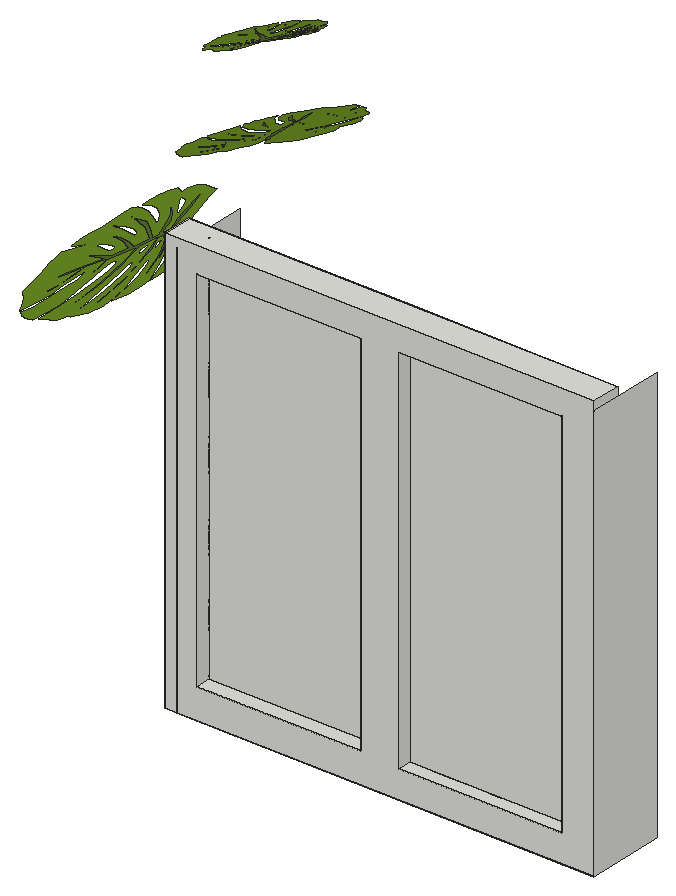
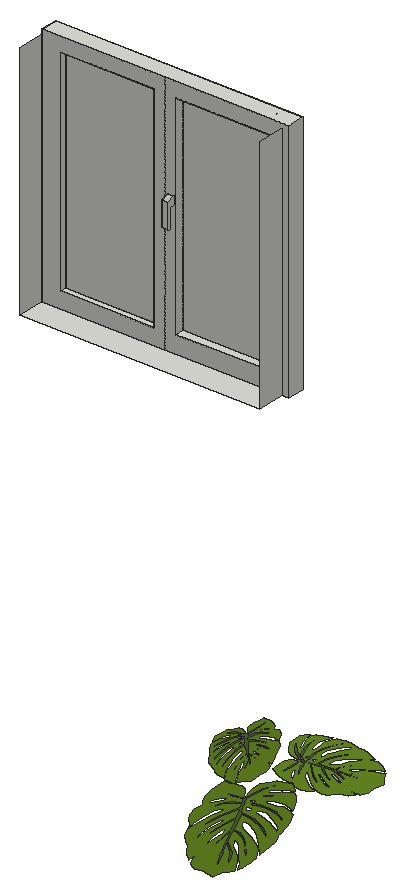
# SketchUp Ruby script. Lengths in inches.
U = 1.inch
M = Sketchup.active_model
def pt(a) = Geom::Point3d.new(a.map { |v| v * U })
def face(e, loops, mat)
  f = e.add_face(loops[0].map { |a| pt(a) })
  loops[1..].each { |l| e.add_face(l.map { |a| pt(a) }).erase! }
  f.material = f.back_material = mat if mat
  f
end
# faces: each face lists its corners as indices into pts; further lists are holes
def faces(e, pts, list, mat = nil) = list.each { |f| face(e, (f[0].is_a?(Array) ? f : [f]).map { |l| l.map { |i| pts[i] } }, mat) }
# xy, xz, yz: faces in a plane at the given z, y or x. An outline is a flat list of corners, or four numbers for a rectangle; further outlines are holes
def ring(l) = l.size == 4 ? [[l[0], l[1]], [l[2], l[1]], [l[2], l[3]], [l[0], l[3]]] : l.each_slice(2).to_a
def flat(e, list, mat, &to3) = list.each { |f| face(e, (f[0].is_a?(Array) ? f : [f]).map { |l| ring(l).map { |u, v| to3.(u, v) } }, mat) }
def xy(e, z, list, mat = nil) = flat(e, list, mat) { |x, y| [x, y, z] }
def xz(e, y, list, mat = nil) = flat(e, list, mat) { |x, z| [x, y, z] }
def yz(e, x, list, mat = nil) = flat(e, list, mat) { |y, z| [x, y, z] }
def lines(e, pts, list) = list.each { |a, b| e.add_line(pt(pts[a]), pt(pts[b])) }
# prism: a flat outline (further loops are holes) pulled along v
def prism(e, loops, v, mat = nil)
  f = face(e, loops, mat); d = Geom::Vector3d.new(v.map { |x| x * U })
  f.pushpull(f.normal.samedirection?(d) ? d.length : -d.length)
end
def box(e, o, s, mat = nil) = prism(e, [[o, [o[0] + s[0], o[1], o[2]], [o[0] + s[0], o[1] + s[1], o[2]], [o[0], o[1] + s[1], o[2]]]], [0, 0, s[2]], mat)
def at(x, y, z, deg = 0) = Geom::Transformation.translation(pt([x, y, z])) * Geom::Transformation.rotation(ORIGIN, Z_AXIS, deg.degrees)
def axes(o, x, y, z) = Geom::Transformation.new([*x, 0, *y, 0, *z, 0, *pt(o).to_a, 1])
def part(name) = M.definitions.add(name)
# library, detail: a bought-in or finely detailed component or shape, given as its bounding box
def library(name, o, s) = part(name).tap { |d| box(d.entities, o, s) }
def detail(e, o, s) = box(e.add_group.entities, o, s)
def put(e, d, t, mat = nil) = e.add_instance(d, t).tap { |i| i.material = mat if mat }
def group(e, t, mat = nil) = e.add_group.tap { |g| g.transformation = t; g.material = mat if mat }.entities
root = M.entities
M.materials.add("[0059_DarkOliveGreen]").color = [85, 107, 47]
M.materials.add("[0061_OliveDrab]").color = [107, 142, 35]
c1 = part("Window")
xy(c1.entities,31.72,[[-0.78,88.6,2.72,128.1]])
xy(c1.entities,34.95,[[-0.78,91.53,0.84,106.59],[0.84,91.53,1.05,97.58],[1.05,91.53,1.42,106.59],[1.42,91.53,2.72,106.59],[0.84,97.58,1.05,98.18],
  [0.84,98.18,1.05,106.59]])
xy(c1.entities,35.27,[[-0.78,110.09,0.97,125.14],[1.05,110.09,2.72,125.14]])
xy(c1.entities,58.35,[[2.72,108.74,3.8,109.74]])
xy(c1.entities,77.8125,[[-0.78,110.09,2.72,125.14],[0.97,110.09,1.05,125.14]])
xy(c1.entities,77.93,[[-0.78,91.53,0.84,106.59],[1.05,91.53,1.42,106.59],[1.42,91.53,2.72,106.59]])
xy(c1.entities,80.72,[[-0.78,88.6,2.72,128.1]])
xz(c1.entities,88.6,[[-0.78,31.72,2.72,80.72]])
xz(c1.entities,91.53,[[-0.78,34.95,0.84,77.93],[1.05,34.95,1.42,77.93],[1.42,34.95,2.72,77.93]])
xz(c1.entities,106.59,[[-0.78,34.95,0.84,77.93],[0.84,34.95,1.05,77.93],[0.84,34.95,2.72,77.93]])
xz(c1.entities,108.74,[[3.8,54.35,4.22,54.6,4.22,59.47,2.72,59.97,2.72,58.35,3.8,58.35]])
xz(c1.entities,109.74,[[3.8,54.35,3.8,58.35,2.72,58.35,2.72,59.97,4.22,59.47,4.22,54.6]])
xz(c1.entities,110.09,[[-0.78,35.27,0.97,77.8125],[1.05,35.27,2.72,77.8125]])
xz(c1.entities,125.14,[[-0.78,35.27,0.97,77.8125],[0.97,35.27,1.05,80.72],[1.05,35.27,2.72,77.8125]])
xz(c1.entities,128.1,[[-0.78,31.72,2.72,80.72]])
yz(c1.entities,-0.78,[[[88.6,31.72,128.1,80.72],[91.53,34.95,106.59,77.93],[110.09,35.27,125.14,77.8125]]])
yz(c1.entities,0.84,[[91.53,34.95,106.59,77.93]])
yz(c1.entities,0.97,[[110.09,35.27,125.14,77.8125]])
yz(c1.entities,1.05,[[91.53,34.95,106.59,77.93],[110.09,35.27,125.14,77.8125]])
yz(c1.entities,1.42,[[91.53,34.95,106.59,77.93]])
yz(c1.entities,2.72,[[[88.6,31.72,108.35,80.72],[91.53,34.95,106.59,77.93]],[[108.35,31.72,128.1,80.72],[110.09,35.27,125.14,77.8125],[108.74,58.35,109.74,59.97]]])
yz(c1.entities,3.8,[[108.74,54.35,109.74,58.35]])
yz(c1.entities,4.22,[[108.74,54.6,109.74,59.47]])
p = [[4.22,108.74,54.6],[3.8,108.74,54.35],[3.8,109.74,54.35],[4.22,109.74,54.6],[2.72,109.74,59.97],[2.72,108.74,59.97],
  [4.22,108.74,59.47],[4.22,109.74,59.47],[-0.78,86.4,89.94],[-0.78,86.44,89.94],[15.22,130.69,89.94],[15.22,130.65,89.94],
  [-0.78,86.44,28.19],[-0.78,86.4,28.19],[7.72,130.69,89.94],[7.72,130.65,89.94]]
faces(c1.entities,p,[[0,1,2,3],[4,5,6,7]])
lines(c1.entities,p,[[8,9],[10,11],[12,13],[14,15]])
xy(root,27.371,[[370.055,0,418.055,9]])
yz(root,370.055,[[0,27.371,9,75.371]])
yz(root,418.055,[[0,27.371,9,75.371]])
p = [[304.853,86.435,19.981],[304.726,87.415,20.148],[303.01,88.008,19.663],[301.981,87.975,19.288],[301.382,87.471,18.965],[301.09,86.892,18.736],
  [300.149,87.468,18.524],[299.286,87.124,18.141],[298.799,86.499,17.832],[298.373,85.322,17.425],[298.178,84.934,17.271],[299.213,84.857,17.624],
  [300.273,84.32,17.887],[301.29,83.488,18.07],[302.026,82.457,18.11],[302.165,82.132,18.089],[302.109,82.02,18.044],[301.858,82.152,17.983],
  [300.655,83.202,17.781],[299.591,83.89,17.55],[298.448,84.458,17.265],[297.836,84.626,17.083],[297.312,84.371,16.84],[297.025,83.789,16.612],
  [296.718,82.818,16.292],[296.461,81.926,16.007],[296.333,81.471,15.862],[295.857,80.704,15.526],[295.523,79.825,15.217],[295.321,78.928,14.95],
  [295.188,78.454,14.8],[295.764,78.52,15.02],[296.637,78.608,15.351],[295.079,77.7,14.598],[294.894,77.446,14.477],[294.84,76.614,14.277],
  [294.786,75.781,14.078],[295.187,73.872,13.807],[295.382,71.16,13.29],[296.346,70.067,13.397],[297.02,68.972,13.401],[297.397,68.268,13.383],
  [298.383,69.632,14.031],[298.919,70.699,14.454],[299.293,72.227,14.918],[299.524,73.307,15.234],[299.788,73.832,15.442],[300.004,74.262,15.612],
  [300.15,74.259,15.664],[300.198,73.971,15.619],[300.086,73.122,15.395],[299.895,72.401,15.171],[299.296,70.915,14.635],[298.749,69.673,14.171],
  [298.449,68.884,13.892],[298.097,68.367,13.655],[297.723,67.985,13.438],[298.306,67.424,13.525],[298.803,67.163,13.646],[299.247,67.023,13.775],
  [299.602,66.96,13.887],[300.017,66.816,14.004],[300.781,68.035,14.542],[301.191,69.196,14.939],[301.38,70.211,15.227],[301.593,72.102,15.712],
  [301.655,73.544,16.047],[301.746,74.764,16.343],[301.872,75.673,16.585],[302.089,76.105,16.757],[302.383,76.132,16.867],[302.51,75.448,16.765],
  [302.585,74.513,16.589],[302.439,72.875,16.182],[302.068,71.113,15.668],[301.485,69.163,15.038],[300.591,66.964,14.242],[302.083,66.72,14.722],
  [302.967,66.685,15.03],[303.354,67.032,15.244],[303.759,67.837,15.5625],[303.993,68.822,15.859],[304.085,70.153,16.18],[304.151,71.285,16.449],
  [304.227,72.957,16.838],[304.177,74.194,17.088],[304.134,75.161,17.282],[304.076,75.633,17.364],[304.212,75.904,17.471],[304.42,75.613,17.483],
  [304.682,74.901,17.422],[304.81,73.776,17.224],[304.701,71.506,16.693],[304.536,70.171,16.345],[304.314,68.979,16.008],[304.105,68.43,15.814],
  [303.763,67.336,15.455],[304.007,67.295,15.534],[304.867,67.564,15.899],[305.631,67.851,16.234],[306.502,68.955,16.784],[306.663,70.115,17.093],
  [306.541,71.968,17.451],[306.178,73.597,17.674],[305.915,75.086,17.903],[305.779,75.738,17.995],[305.805,76.106,18.084],[305.959,76.0625,18.13],
  [306.284,75.309,18.083],[306.736,73.486,17.849],[306.87,72.009,17.577],[306.863,69.648,17.064],[307.894,70.835,17.689],[308.435,72.034,18.142],
  [308.524,73.041,18.392],[308.351,73.56,18.442],[307.78,75.125,18.577],[307.255,76.282,18.64],[306.924,77.194,18.719],[306.885,77.558,18.784],
  [307.028,77.672,18.86],[307.17,77.473,18.868],[307.863,76.019,18.8],[308.26,74.845,18.688],[308.517,73.801,18.554],[308.692,73.011,18.445],
  [309.07,73.983,18.791],[309.185,74.891,19.028],[309.023,76.065,19.225],[308.6875,77.165,19.343],[308.457,78.286,19.503],[308.039,78.87,19.481],
  [307.531,79.84,19.509],[306.939,80.668,19.477],[306.154,81.0625,19.282],[305.336,80.946,18.965],[304.862,80.663,18.734],[304.685,81.227,18.793],
  [305.078,81.701,19.036],[305.479,82.498,19.352],[305.452,83.538,19.567],[305.152,85.05,19.788],[303.837,83.57,18.998],[303.602,86.415,19.53],
  [303.935,84.587,19.253],[304.633,80.764,18.674],[305.238,80.297,18.789],[306.537,79.556,19.093],[307.35,78.587,19.173],[307.821,77.747,19.159],
  [306.459,79.052,18.956],[305.334,79.816,18.719],[304.704,80.055,18.546],[305.709,78.983,18.673],[306.658,76.874,18.555],[307.16,75.186,18.369],
  [307.55,73.447,18.132],[307.667,72.574,17.985],[306.882,75.265,18.287],[306.326,76.863,18.434],[305.574,78.624,18.547],[304.92,79.538,18.511],
  [304.553,79.914,18.462],[304.325,79.824,18.36],[304.274,79.534,18.28],[304.494,78.754,18.189],[304.849,77.972,18.147],[305.083,77.047,18.03],
  [305.535,74.371,17.612],[305.678,72.658,17.292],[305.547,71.055,16.898],[305.461,69.756,16.586],[305.214,69.265,16.391],[305.391,71.771,16.997],
  [305.336,73.187,17.285],[305.081,75.424,17.678],[304.655,77.399,17.953],[304.067,79.561,18.211],[303.143,78.435,17.637],[303.364,76.766,17.355],
  [303.545,75.193,17.079],[303.371,71.93,16.31],[303.047,70.316,15.845],[302.762,69.236,15.509],[302.508,68.731,15.309],[302.814,70.26,15.75],
  [303.085,72.777,16.392],[303.17,75.999,17.12],[302.89,77.932,17.438],[301.118,76.205,16.431],[301.248,74.907,16.197],[301.067,73.32,15.788],
  [300.677,71.795,15.318],[300.257,70.645,14.92],[299.623,69.385,14.42],[300.519,71.996,15.306],[300.883,73.507,15.763],[301.002,74.914,16.11],
  [300.91,76.187,16.353],[299.529,75.091,15.623],[299.279,73.692,15.23],[298.851,72.441,14.806],[298.336,71.418,14.401],[297.833,70.966,14.123],
  [298.696,72.681,14.803],[299.039,73.967,15.204],[299.24,75,15.499],[298.169,73.938,14.887],[297.593,73.382,14.561],[296.862,72.584,14.127],
  [296.957,72.727,14.192],[298.035,74.268,14.91],[299.134,75.494,15.568],[300.444,76.423,16.238],[297.347,77.051,15.267],[300.877,77.043,16.526],
  [301.929,78.144,17.141],[300.413,79.14,16.815],[297.956,80.158,16.158],[299.766,79.792,16.725],[301.436,79.043,17.159],[302.316,78.435,17.342],
  [303.194,79.514,17.89],[301.286,81.263,17.586],[298.505,82.99,16.967],[300.734,82.283,17.61],[302.209,81.07,17.874],[303.465,79.733,18.034],
  [303.829,80.089,18.241],[303.328,81.434,18.353],[302.667,83.224,18.505],[301.159,85.023,18.355],[302.513,83.794,18.573],[303.521,82.384,18.628],
  [303.913,80.793,18.423],[304.096,80.536,18.433],[304.359,81.057,18.64],[299.918,81.263,17.098],[300.941,80.666,17.334],[301.194,80.354,17.357],
  [301.251,80.133,17.329],[301.134,80.043,17.268],[300.725,80.221,17.16],[299.749,80.657,16.906],[298.671,81.125,16.623],[297.537,81.486,16.296],
  [297.004,81.674,16.146],[298.616,81.621,16.711],[300.042,78.487,16.541],[300.406,78.202,16.61],[300.43,77.879,16.548],[300.268,77.702,16.452],
  [299.907,77.673,16.316],[299.623,77.789,16.24],[298.485,78.208,15.924],[297.431,78.608,15.634],[299.046,78.667,16.224],[302.614,85.525,18.984],
  [303.065,84.728,18.972],[303.322,84.025,18.912],[303.298,83.648,18.822],[303.179,83.529,18.754],[302.408,84.7,18.732],[301.802,85.741,18.741],
  [301.686,86.044,18.765],[302.124,86.019,18.916],[304.154,78.157,17.939],[304.194,77.552,17.822],[304.057,77.098,17.675],[303.865,77.141,17.615],
  [303.658,77.717,17.666],[303.704,78.417,17.834],[303.93,78.638,17.963],[304.914,79.202,18.436],[305.072,78.578,18.358],[305.078,78.113,18.259],
  [304.882,78.133,18.193],[304.715,78.808,18.28],[304.698,79.303,18.381],[306.194,103.112,20.08],[306.543,104.665,19.869],[306.335,106.088,19.486],
  [305.956,106.891,19.177],[305.242,107.593,18.77],[305.007,107.915,18.616],[304.961,106.209,18.969],[304.635,104.461,19.231],[304.13,102.783,19.414],
  [303.506,101.568,19.454],[303.308,101.338,19.434],[303.24,101.431,19.389],[303.32,101.846,19.328],[303.957,103.83,19.126],[304.374,105.584,18.895],
  [304.719,107.47,18.609],[304.821,108.479,18.427],[304.666,109.344,18.185],[304.313,109.817,17.956],[303.725,110.323,17.636],[303.184,110.747,17.352],
  [302.908,110.959,17.207],[302.443,111.744,16.871],[301.91,112.294,16.561],[301.366,112.628,16.295],[301.079,112.847,16.145],[301.119,111.897,16.365],
  [301.172,110.457,16.696],[300.621,113.027,15.942],[300.468,113.332,15.821],[299.963,113.421,15.622],[299.458,113.51,15.422],[298.301,112.849,15.152],
  [296.657,112.527,14.634],[295.994,110.937,14.742],[295.33,109.825,14.746],[294.903,109.204,14.728],[295.73,107.578,15.375],[296.377,106.692,15.798],
  [297.303,106.077,16.262],[297.958,105.696,16.579],[298.277,105.26,16.787],[298.537,104.903,16.957],[298.536,104.663,17.009],[298.361,104.584,16.963],
  [297.846,104.769,16.739],[297.409,105.083,16.515],[296.508,106.071,15.98],[295.755,106.973,15.515],[295.277,107.468,15.237],[294.964,108.049,14.999],
  [294.732,108.665,14.783],[294.392,107.704,14.87],[294.234,106.885,14.991],[294.149,106.151,15.119],[294.111,105.567,15.232],[294.023,104.883,15.349],
  [294.762,103.622,15.886],[295.466,102.945,16.284],[296.081,102.634,16.571],[297.228,102.282,17.057],[298.102,102.18,17.391],[298.842,102.031,17.688],
  [299.392,101.823,17.93],[299.655,101.464,18.101],[299.671,100.98,18.212],[299.256,100.77,18.109],[298.69,100.646,17.934],[297.696,100.887,17.527],
  [296.628,101.499,17.013],[295.446,102.46,16.382],[294.113,103.935,15.586],[293.965,101.474,16.066],[293.944,100.015,16.375],[294.154,99.377,16.588],
  [294.642,98.709,16.907],[295.239,98.323,17.204],[296.046,98.173,17.525],[296.733,98.064,17.794],[297.746,97.938,18.183],[298.496,98.02,18.433],
  [299.082,98.092,18.627],[299.369,98.186,18.709],[299.533,97.962,18.816],[299.357,97.619,18.827],[298.925,97.187,18.767],[298.243,96.976,18.569],
  [296.866,97.156,18.038],[296.057,97.428,17.69],[295.334,97.794,17.353],[295.001,98.139,17.159],[294.339,98.704,16.8],[294.313,98.3,16.878],
  [294.477,96.882,17.244],[294.65,95.622,17.579],[295.32,94.185,18.129],[296.023,93.919,18.438],[297.147,94.121,18.795],[298.134,94.719,19.019],
  [299.037,95.153,19.247],[299.432,95.378,19.34],[299.655,95.335,19.429],[299.629,95.081,19.474],[299.172,94.545,19.427],[298.067,93.799,19.194],
  [297.171,93.578,18.922],[295.74,93.589,18.408],[296.459,91.889,19.033],[297.187,90.997,19.486],[297.797,90.85,19.736],[298.112,91.136,19.787],
  [299.06,92.077,19.922],[299.762,92.943,19.985],[300.315,93.49,20.064],[300.536,93.554,20.129],[300.605,93.317,20.205],[300.484,93.083,20.213],
  [299.602,91.94,20.145],[298.891,91.286,20.032],[298.258,90.862,19.898],[297.779,90.572,19.79],[298.368,89.949,20.135],[298.919,89.76,20.373],
  [299.63,90.026,20.57],[300.297,90.58,20.688],[300.977,90.961,20.848],[301.331,91.65,20.825],[301.919,92.488,20.854],[302.421,93.464,20.822],
  [302.66,94.76,20.627],[302.589,96.109,20.309],[302.418,96.891,20.079],[302.76,97.182,20.138],[303.047,96.534,20.381],[303.53,95.873,20.696],
  [304.161,95.918,20.912],[305.077,96.413,21.132],[305.917,96.904,21.326],[306.511,97.114,21.492],[306.871,99.945,21.008],[306.851,101.643,20.633],
  [306.546,102.631,20.31],[303.829,107.376,18.312],[303.4,103.7,18.955],[302.665,101.267,19.219],[301.854,99.194,19.378],[302.07,98.594,19.586],
  [302.885,99.421,19.698],[303.971,100.511,19.849],[305.061,102.999,19.7],[304.316,100.764,19.918],[303.461,99.102,19.973],[302.496,98.455,19.768],
  [302.341,98.153,19.778],[302.657,97.721,19.984],[304.18,98.581,20.342],[305.905,98.969,20.874],[302.479,97.268,20.019],[302.196,96.27,20.134],
  [301.747,94.127,20.4375],[301.159,92.786,20.518],[300.65,92.01,20.504],[301.441,94.257,20.3],[301.904,96.113,20.064],[302.049,97.152,19.89],
  [301.399,95.493,20.018],[300.121,93.928,19.9],[299.097,93.099,19.714],[298.043,92.457,19.476],[297.514,92.263,19.329],[299.145,93.559,19.631],
  [300.114,94.475,19.779],[301.181,95.716,19.891],[301.736,96.794,19.856],[301.964,97.399,19.806],[301.909,97.776,19.705],[301.733,97.86,19.624],
  [301.26,97.497,19.534],[300.787,96.912,19.491],[300.226,96.526,19.375],[298.603,95.781,18.956],[297.565,95.544,18.637],[296.593,95.761,18.243],
  [295.805,95.903,17.931],[295.508,96.31,17.736],[297.027,96.017,18.342],[297.886,96.108,18.629],[299.242,96.53,19.022],[300.439,97.232,19.298],
  [301.75,98.202,19.556],[301.067,99.726,18.982],[300.055,99.361,18.7],[299.102,99.0625,18.424],[297.124,99.35,17.655],[296.145,99.885,17.189],
  [295.49,100.354,16.854],[295.184,100.773,16.654],[296.111,100.269,17.094],[297.637,99.821,17.736],[299.591,99.682,18.464],[300.762,100.144,18.783],
  [299.715,103.066,17.776],[298.928,102.851,17.541],[297.966,103.15,17.133],[297.041,103.794,16.663],[296.345,104.486,16.264],[295.581,105.532,15.765],
  [297.163,104.054,16.65],[298.079,103.454,17.107],[298.932,103.257,17.455],[299.704,103.409,17.698],[299.04,105.687,16.967],[298.191,106.099,16.575],
  [297.434,106.806,16.151],[296.813,107.655,15.745],[296.539,108.484,15.468],[297.579,107.062,16.147],[298.359,106.496,16.549],[298.985,106.165,16.844],
  [298.341,107.93,16.232],[298.004,108.88,15.905],[297.52,110.086,15.471],[297.606,109.929,15.536],[298.541,108.151,16.255],[299.284,106.339,16.913],
  [299.847,104.177,17.582],[300.228,109.286,16.612],[300.223,103.464,17.871],[300.891,101.728,18.486],[301.495,104.229,18.16],[302.112,108.281,17.503],
  [301.89,105.296,18.07],[301.436,102.542,18.504],[301.067,101.089,18.687],[301.721,99.641,19.234],[302.781,102.789,18.931],[302.781,105.046,18.442],
  [302.42,103.357,18.679],[302.23,102.941,18.701],[302.097,102.847,18.674],[302.042,103.04,18.613],[302.15,103.715,18.505],[302.414,105.325,18.251],
  [302.698,107.102,17.967],[302.917,108.972,17.641],[303.031,109.852,17.491],[302.999,107.192,18.055],[301.099,104.841,17.886],[300.926,104.24,17.954],
  [300.73,104.201,17.893],[300.622,104.467,17.797],[300.605,105.064,17.661],[300.675,105.532,17.585],[300.93,107.41,17.269],[301.172,109.148,16.979],
  [301.208,106.484,17.569],[305.665,101.407,20.261],[305.366,100.598,20.329],[304.882,99.855,20.317],[304.456,99.431,20.257],[304.227,99.47,20.166],
  [304.155,99.666,20.098],[304.865,100.938,20.076],[305.496,101.938,20.085],[305.68,102.128,20.11],[300.282,98.536,18.96],[300.632,98.877,19.011],
  [301.056,98.8,19.179],[301.19,98.428,19.307],[300.899,98.058,19.283],[300.532,97.992,19.166],[300.257,98.218,19.019],[301.532,96.805,19.781],
  [301.154,96.544,19.702],[300.872,96.534,19.604],[300.884,96.857,19.538],[301.294,97.132,19.625],[301.593,97.161,19.726],[303.029,92.514,31.743],
  [302.945,91.868,31.853],[301.8125,91.477,31.533],[301.133,91.498,31.286],[300.738,91.831,31.073],[300.545,92.213,30.921],[299.924,91.833,30.782],
  [299.354,92.06,30.529],[299.033,92.473,30.325],[298.752,93.249,30.056],[298.623,93.506,29.955],[299.306,93.556,30.188],[300.006,93.911,30.361],
  [300.677,94.46,30.482],[301.163,95.14,30.508],[301.255,95.355,30.494],[301.218,95.429,30.465],[301.052,95.342,30.425],[300.258,94.649,30.291],
  [299.556,94.194,30.139],[298.801,93.819,29.95],[298.398,93.709,29.83],[298.052,93.877,29.67],[297.862,94.261,29.519],[297.66,94.902,29.308],
  [297.49,95.49,29.12],[297.405,95.791,29.025],[297.091,96.297,28.803],[296.871,96.877,28.599],[296.738,97.469,28.423],[296.65,97.782,28.324],
  [297.03,97.738,28.469],[297.606,97.681,28.687],[296.578,98.28,28.19],[296.456,98.447,28.11],[296.42,98.997,27.979],[296.385,99.546,27.847],
  [296.649,100.806,27.668],[296.778,102.596,27.327],[297.414,103.317,27.398],[297.859,104.041,27.4],[298.108,104.505,27.388],[298.758,103.605,27.816],
  [299.113,102.9,28.095],[299.359,101.892,28.401],[299.511,101.179,28.61],[299.686,100.833,28.748],[299.828,100.549,28.86],[299.925,100.551,28.894],
  [299.956,100.741,28.864],[299.882,101.301,28.716],[299.757,101.777,28.568],[299.361,102.758,28.215],[299,103.578,27.908],[298.802,104.098,27.725],
  [298.57,104.439,27.568],[298.323,104.692,27.425],[298.708,105.062,27.482],[299.036,105.234,27.562],[299.329,105.327,27.647],[299.563,105.368,27.721],
  [299.837,105.464,27.799],[300.341,104.659,28.153],[300.612,103.893,28.416],[300.737,103.223,28.605],[300.877,101.975,28.926],[300.918,101.023,29.147],
  [300.978,100.218,29.342],[301.061,99.618,29.502],[301.205,99.332,29.615],[301.398,99.314,29.688],[301.482,99.766,29.62],[301.532,100.383,29.504],
  [301.435,101.464,29.236],[301.191,102.627,28.896],[300.806,103.914,28.48],[300.216,105.366,27.955],[301.2,105.527,28.272],[301.784,105.55,28.476],
  [302.04,105.32,28.616],[302.307,104.789,28.827],[302.461,104.139,29.023],[302.522,103.261,29.235],[302.565,102.514,29.412],[302.616,101.41,29.669],
  [302.583,100.594,29.834],[302.554,99.956,29.962],[302.516,99.644,30.016],[302.606,99.465,30.087],[302.743,99.657,30.094],[302.916,100.127,30.054],
  [303,100.87,29.924],[302.928,102.368,29.573],[302.82,103.249,29.344],[302.673,104.036,29.121],[302.535,104.398,28.993],[302.309,105.12,28.756],
  [302.47,105.147,28.808],[303.038,104.969,29.049],[303.542,104.78,29.27],[304.117,104.051,29.633],[304.223,103.286,29.837],[304.143,102.063,30.073],
  [303.903,100.988,30.22],[303.73,100.005,30.371],[303.64,99.575,30.432],[303.657,99.332,30.491],[303.759,99.361,30.521],[303.973,99.858,30.49],
  [304.272,101.061,30.336],[304.36,102.036,30.157],[304.356,103.594,29.818],[305.036,102.811,30.23],[305.393,102.019,30.529],[305.452,101.354,30.694],
  [305.337,101.012,30.727],[304.96,99.98,30.816],[304.614,99.216,30.858],[304.395,98.614,30.91],[304.37,98.373,30.953],[304.464,98.298,31.003],
  [304.558,98.429,31.008],[305.016,99.39,30.964],[305.277,100.164,30.89],[305.447,100.853,30.801],[305.563,101.375,30.729],[305.812,100.733,30.958],
  [305.888,100.134,31.114],[305.781,99.359,31.244],[305.56,98.633,31.322],[305.407,97.893,31.428],[305.131,97.508,31.413],[304.796,96.867,31.432],
  [304.406,96.321,31.411],[303.887,96.061,31.282],[303.347,96.138,31.072],[303.035,96.324,30.92],[302.918,95.952,30.959],[303.177,95.639,31.119],
  [303.442,95.113,31.328],[303.424,94.426,31.47],[303.226,93.429,31.615],[302.358,94.406,31.094],[302.203,92.528,31.445],[302.423,93.734,31.263],
  [302.884,96.257,30.881],[303.283,96.566,30.956],[304.14,97.055,31.157],[304.677,97.695,31.21],[304.987,98.249,31.201],[304.088,97.388,31.066],
  [303.346,96.884,30.91],[302.93,96.726,30.796],[303.594,97.433,30.88],[304.22,98.825,30.802],[304.552,99.939,30.679],[304.809,101.087,30.523],
  [304.886,101.663,30.425],[304.368,99.887,30.625],[304.001,98.832,30.722],[303.504,97.67,30.796],[303.073,97.067,30.773],[302.831,96.818,30.74],
  [302.68,96.878,30.674],[302.647,97.07,30.62],[302.792,97.584,30.561],[303.026,98.1,30.532],[303.181,98.711,30.455],[303.479,100.477,30.179],
  [303.573,101.608,29.968],[303.487,102.666,29.708],[303.43,103.523,29.502],[303.267,103.847,29.374],[303.384,102.193,29.774],[303.348,101.258,29.963],
  [303.179,99.782,30.223],[302.898,98.478,30.405],[302.51,97.052,30.575],[301.9,97.795,30.196],[302.046,98.897,30.01],[302.165,99.934,29.828],
  [302.051,102.088,29.32],[301.836,103.153,29.013],[301.649,103.866,28.792],[301.481,104.199,28.66],[301.683,103.19,28.95],[301.862,101.529,29.374],
  [301.918,99.402,29.855],[301.733,98.127,30.065],[300.564,99.266,29.4],[300.65,100.123,29.245],[300.53,101.17,28.976],[300.272,102.177,28.666],
  [299.995,102.936,28.403],[299.577,103.768,28.073],[300.168,102.045,28.657],[300.408,101.047,28.959],[300.487,100.119,29.188],[300.426,99.278,29.349],
  [299.515,100.002,28.867],[299.35,100.925,28.608],[299.067,101.751,28.328],[298.727,102.426,28.06],[298.396,102.725,27.877],[298.965,101.593,28.325],
  [299.191,100.743,28.59],[299.324,100.062,28.785],[298.617,100.763,28.381],[298.237,101.13,28.166],[297.755,101.657,27.879],[297.818,101.562,27.922],
  [298.529,100.545,28.397],[299.254,99.736,28.831],[300.119,99.123,29.273],[298.075,98.708,28.632],[300.404,98.714,29.463],[301.099,97.987,29.869],
  [300.098,97.329,29.653],[298.477,96.658,29.22],[299.671,96.899,29.594],[300.773,97.393,29.881],[301.355,97.795,30.001],[301.934,97.083,30.363],
  [300.674,95.929,30.163],[298.839,94.788,29.754],[300.31,95.255,30.178],[301.284,96.056,30.353],[302.113,96.938,30.458],[302.353,96.703,30.595],
  [302.022,95.815,30.669],[301.586,94.634,30.769],[300.591,93.447,30.67],[301.485,94.258,30.814],[302.15,95.189,30.85],[302.408,96.239,30.715],
  [302.529,96.408,30.722],[302.702,96.064,30.858],[299.771,95.928,29.84],[300.447,96.322,29.996],[300.614,96.528,30.011],[300.651,96.674,29.993],
  [300.574,96.733,29.953],[300.304,96.616,29.882],[299.66,96.328,29.714],[298.949,96.019,29.527],[298.2,95.781,29.311],[297.848,95.657,29.212],
  [298.913,95.692,29.585],[299.853,97.76,29.473],[300.094,97.948,29.518],[300.109,98.162,29.477],[300.003,98.279,29.414],[299.764,98.297,29.325],
  [299.577,98.221,29.274],[298.826,97.944,29.066],[298.13,97.68,28.874],[299.196,97.642,29.264],[301.551,93.115,31.085],[301.848,93.642,31.077],
  [302.018,94.105,31.038],[302.002,94.354,30.978],[301.924,94.433,30.933],[301.415,93.66,30.919],[301.015,92.973,30.924],[300.939,92.773,30.941],
  [301.227,92.789,31.04],[302.568,97.978,30.395],[302.594,98.377,30.318],[302.503,98.677,30.221],[302.376,98.649,30.182],[302.24,98.269,30.215],
  [302.27,97.807,30.326],[302.42,97.661,30.411],[303.069,97.288,30.724],[303.173,97.7,30.672],[303.177,98.007,30.607],[303.048,97.994,30.563],
  [302.938,97.548,30.621],[302.926,97.222,30.687],[298.761,89.162,25.941],[298.759,89.158,25.94]]
faces(root,p,[[[0,1,2,3,4,5,6,7,8,9,10,11,12,13,14,15,16,17,18,19,20,21,22,23,24,25,26,27,28,29,30,31,32,33,34,35,36,37,38,39,40,41,42,43,44,45,46,47,48,49,50,51,52,53,54,55,56,57,58,59,60,61,62,63,64,65,66,67,68,69,70,71,72,73,74,75,76,77,78,79,80,81,82,83,84,85,86,87,88,89,90,91,92,93,94,95,80,96,97,98,99,100,101,102,103,104,105,106,107,108,109,110,111,112,113,114,115,116,117,118,119,120,121,122,123,124,125,126,127,128,129,130,131,132,133,134,135,136,137,138,139,140,141],[142,143,144,145,146,147,148,149,150,151,152,153,154,155,156,157,158,159,160,161,162,163,164,165,166,167,168,169,170,171,172,173,174,175,176,177,178,179,180,181,182,183,184,185,186,187,188,189,190,191,192,193,194,195,196,197,198,199,200,201,202,203,204,205,206,207,208,209,210,211,212,213,214,215,216,217,218,219,220,221,222,223,224,225,226,227,228,229,230,231,232,233,234,235,236],[237,238,239,240,241,242,243,244,245,246,247],[248,249,250,251,252,253,254,255,256],[257,258,259,260,261,262,263,264,265],[266,267,268,269,270,271,272],[273,274,275,276,277,278]],[[279,280,281,282,283,284,285,286,287,288,289,290,291,292,293,294,295,296,297,298,299,300,301,302,303,304,305,306,307,308,309,310,311,312,313,314,315,316,317,318,319,320,321,322,323,324,325,326,327,328,329,330,331,332,333,334,335,336,337,338,339,340,341,342,343,344,345,346,347,348,349,350,351,352,353,354,355,356,357,358,359,360,361,362,363,364,365,366,367,368,369,354,370,371,372,373,374,375,376,377,378,379,380,381,382,383,384,385,386,387,388,389,390,391,392,393,394,395,396,397,398,399,400,401,402,403,404,405,406,407,408,409,410,411,412,413,414,415,416,417,418,419,420],[421,422,423,424,425,426,427,428,429,430,431,432,433,434,435,436,437,438,439,440,441,442,443,444,445,446,447,448,449,450,451,452,453,454,455,456,457,458,459,460,461,462,463,464,465,466,467,468,469,470,471,472,473,474,475,476,477,478,479,480,481,482,483,484,485,486,487,488,489,490,491,492,493,494,495,496,497,498,499,500,501,502,503,504,505,506,507,508,509,510,511,512,513,514],[515,516,517,518,519,520,521,522,523,524,525],[526,527,528,529,530,531,532,533,534],[535,536,537,538,539,540,541,542,543],[544,545,546,547,548,549,550],[551,552,553,554,555,556]],[[557,558,559,560,561,562,563,564,565,566,567,568,569,570,571,572,573,574,575,576,577,578,579,580,581,582,583,584,585,586,587,588,589,590,591,592,593,594,595,596,597,598,599,600,601,602,603,604,605,606,607,608,609,610,611,612,613,614,615,616,617,618,619,620,621,622,623,624,625,626,627,628,629,630,631,632,633,634,635,636,637,638,639,640,641,642,643,644,645,646,647,648,649,650,651,652,637,653,654,655,656,657,658,659,660,661,662,663,664,665,666,667,668,669,670,671,672,673,674,675,676,677,678,679,680,681,682,683,684,685,686,687,688,689,690,691,692,693,694,695,696,697,698],[699,700,701,702,703,704,705,706,707,708,709,710,711,712,713,714,715,716,717,718,719,720,721,722,723,724,725,726,727,728,729,730,731,732,733,734,735,736,737,738,739,740,741,742,743,744,745,746,747,748,749,750,751,752,753,754,755,756,757,758,759,760,761,762,763,764,765,766,767,768,769,770,771,772,773,774,775,776,777,778,779,780,781,782,783,784,785,786,787,788,789,790,791,792,793],[794,795,796,797,798,799,800,801,802,803,804],[805,806,807,808,809,810,811,812,813],[814,815,816,817,818,819,820,821,822],[823,824,825,826,827,828,829],[830,831,832,833,834,835]]],"[0061_OliveDrab]")
faces(root,p,[[143,142,236,235,234,233,232,231,230,229,228,227,226,225,224,223,222,221,220,219,218,217,216,215,214,213,212,211,210,209,208,207,206,205,204,203,202,201,200,199,198,197,196,195,194,193,192,191,190,189,188,187,186,185,184,183,182,181,180,179,178,177,176,175,174,173,172,171,170,169,168,167,166,165,164,163,162,161,160,159,158,157,156,155,154,153,152,151,150,149,148,147,146,145,144],[422,421,514,513,512,511,510,509,508,507,506,505,504,503,502,501,500,499,498,497,496,495,494,493,492,491,490,489,488,487,486,485,484,483,482,481,480,479,478,477,476,475,474,473,472,471,470,469,468,467,466,465,464,463,462,461,460,459,458,457,456,455,454,453,452,451,450,449,448,447,446,445,444,443,442,441,440,439,438,437,436,435,434,433,432,431,430,429,428,427,426,425,424,423],[700,699,793,792,791,790,789,788,787,786,785,784,783,782,781,780,779,778,777,776,775,774,773,772,771,770,769,768,767,766,765,764,763,762,761,760,759,758,757,756,755,754,753,752,751,750,749,748,747,746,745,744,743,742,741,740,739,738,737,736,735,734,733,732,731,730,729,728,727,726,725,724,723,722,721,720,719,718,717,716,715,714,713,712,711,710,709,708,707,706,705,704,703,702,701]],"[0059_DarkOliveGreen]")
lines(root,p,[[836,837]])
put(root,c1,axes([528.8,0.78,-4.35],[0,1,0],[-1.25,0,0],[0,0,1]))
